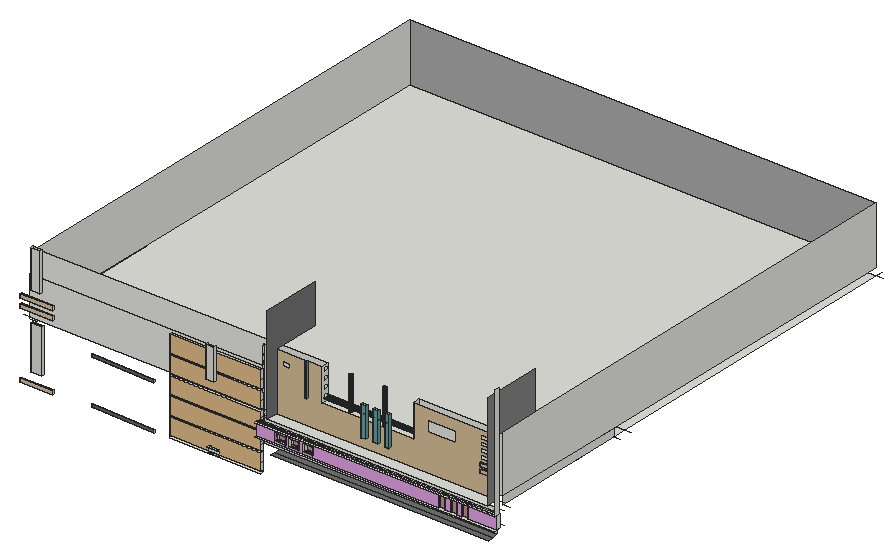
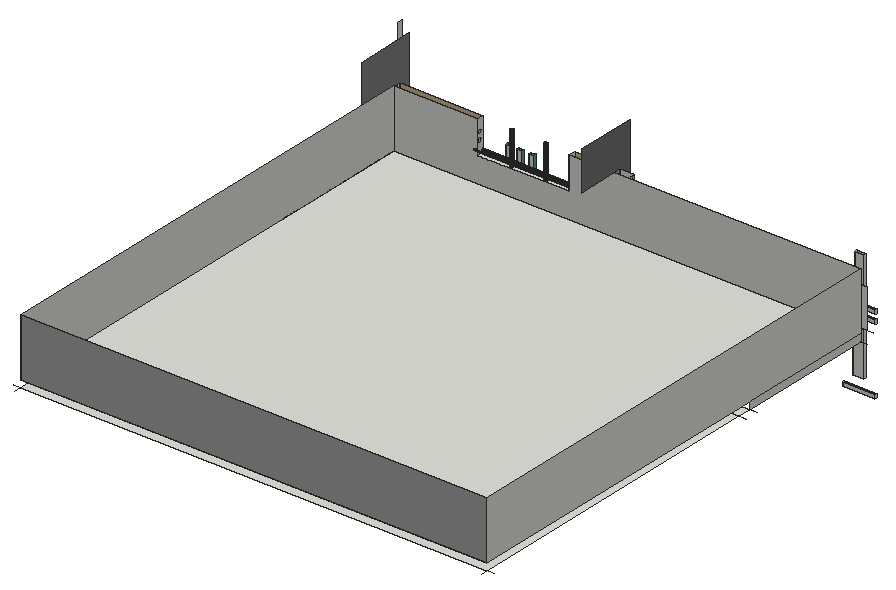
# SketchUp Ruby script. Lengths in inches.
U = 1.inch
M = Sketchup.active_model
def pt(a) = Geom::Point3d.new(a.map { |v| v * U })
def face(e, loops, mat)
  f = e.add_face(loops[0].map { |a| pt(a) })
  loops[1..].each { |l| e.add_face(l.map { |a| pt(a) }).erase! }
  f.material = f.back_material = mat if mat
  f
end
# faces: each face lists its corners as indices into pts; further lists are holes
def faces(e, pts, list, mat = nil) = list.each { |f| face(e, (f[0].is_a?(Array) ? f : [f]).map { |l| l.map { |i| pts[i] } }, mat) }
# xy, xz, yz: faces in a plane at the given z, y or x. An outline is a flat list of corners, or four numbers for a rectangle; further outlines are holes
def ring(l) = l.size == 4 ? [[l[0], l[1]], [l[2], l[1]], [l[2], l[3]], [l[0], l[3]]] : l.each_slice(2).to_a
def flat(e, list, mat, &to3) = list.each { |f| face(e, (f[0].is_a?(Array) ? f : [f]).map { |l| ring(l).map { |u, v| to3.(u, v) } }, mat) }
def xy(e, z, list, mat = nil) = flat(e, list, mat) { |x, y| [x, y, z] }
def xz(e, y, list, mat = nil) = flat(e, list, mat) { |x, z| [x, y, z] }
def yz(e, x, list, mat = nil) = flat(e, list, mat) { |y, z| [x, y, z] }
def lines(e, pts, list) = list.each { |a, b| e.add_line(pt(pts[a]), pt(pts[b])) }
# prism: a flat outline (further loops are holes) pulled along v
def prism(e, loops, v, mat = nil)
  f = face(e, loops, mat); d = Geom::Vector3d.new(v.map { |x| x * U })
  f.pushpull(f.normal.samedirection?(d) ? d.length : -d.length)
end
def box(e, o, s, mat = nil) = prism(e, [[o, [o[0] + s[0], o[1], o[2]], [o[0] + s[0], o[1] + s[1], o[2]], [o[0], o[1] + s[1], o[2]]]], [0, 0, s[2]], mat)
def at(x, y, z, deg = 0) = Geom::Transformation.translation(pt([x, y, z])) * Geom::Transformation.rotation(ORIGIN, Z_AXIS, deg.degrees)
def axes(o, x, y, z) = Geom::Transformation.new([*x, 0, *y, 0, *z, 0, *pt(o).to_a, 1])
def part(name) = M.definitions.add(name)
# library, detail: a bought-in or finely detailed component or shape, given as its bounding box
def library(name, o, s) = part(name).tap { |d| box(d.entities, o, s) }
def detail(e, o, s) = box(e.add_group.entities, o, s)
def put(e, d, t, mat = nil) = e.add_instance(d, t).tap { |i| i.material = mat if mat }
def group(e, t, mat = nil) = e.add_group.tap { |g| g.transformation = t; g.material = mat if mat }.entities
root = M.entities
M.materials.add("[0036_BurlyWood]").color = [222, 184, 135]
M.materials.add("[0042_Sienna]").color = [160, 82, 45]
M.materials.add("[0081_CadetBlue]").color = [95, 158, 160]
M.materials.add("[0119_RosyBrown]").color = [188, 143, 143]
M.materials.add("[0125_Plum]").color = [221, 160, 221]
M.materials.add("[0132_LightGray]").color = [169, 169, 169]
M.materials.add("[0133_Gray]").color = [128, 128, 128]
M.materials.add("[0134_DimGray]").color = [105, 105, 105]
M.materials.add("[Color M05]").color = [114, 114, 114]
M.materials.add("[Formica Beige]").color = [211, 187, 149]
M.materials.add("[Formica Laminate Light]").color = [213, 189, 164]
M.materials.add("[Terrazzo Tile Light]").color = [219, 217, 210]
xy(root,174.63,[[146.81,142.49,186.87,144.49]])
xy(root,178.5,[[332.83,142.31,447.24,145.31]])
xy(root,178.94,[[315.8,139.31,236.15,142.31,236.1875,143.31,315.83,140.31]])
xy(root,179.19,[[146.81,142.49,186.87,144.49]])
xy(root,180.89,[[332.83,142.31,447.24,145.31]])
xy(root,181.94,[[315.8,139.31,315.83,140.31,236.1875,143.31,236.15,142.31]])
xy(root,186.75,[[382.48,139.31,394.98,142.31]])
xy(root,191.55,[[160.7,141.49,173.95,144.49]])
xy(root,200,[[630.77,325.1,694.77,328.1]])
xy(root,201.5625,[[332.83,142.31,447.24,145.31]])
xy(root,203.95,[[332.83,142.31,447.24,145.31]])
xy(root,204,[[626.77,325.1,698.77,328.1]])
xy(root,210.6875,[[467.92,131.81,739.66,137.81],[467.92,137.81,467.92,146.81,737.81,146.81,739.66,137.81]],"[Color M05]")
xy(root,217.49,[[452.48,325.1,494.34,328.1],[494.34,325.1,497.5,328.1],[497.5,325.1,522.78,328.1],[522.78,325.1,525.94,328.1],[525.94,325.1,552.97,328.1],
  [552.97,325.1,556.13,328.1],[556.13,325.1,577.62,328.1]])
xy(root,222.93,[[447.04,325.1,583.06,328.1]])
xy(root,223.5,[[447.24,131.81,746.74,131.81,746.74,134.81,710.41,134.81,710.41,136.81,703.03,136.81,703.03,134.81,696.72,134.81,696.72,136.81,689.35,136.81,689.35,134.81,682.28,134.81,682.28,136.81,674.91,136.81,674.91,134.81,447.24,134.81],[746.74,131.81,746.81,134.81],[682.28,134.81,689.35,137.81],[696.72,134.81,703.03,137.81],[710.41,134.81,746.74,137.81],
  [746.74,134.81,746.81,137.81],[674.91,136.81,682.28,137.81],[689.35,136.81,696.72,137.81],[703.03,136.81,710.41,137.81],[674.91,137.81,682.28,139.81],
  [682.28,137.81,689.35,139.81],[689.35,137.81,696.72,139.81],[696.72,137.81,703.03,139.81],[703.03,137.81,710.41,139.81],[710.41,137.81,746.74,139.81],
  [746.74,137.81,746.81,139.81]])
xy(root,224.625,[[332.83,142.31,447.24,145.31]])
xy(root,225.72,[[470.47,134.81,483.6,137.81],[470.47,137.81,483.6,139.81]])
xy(root,225.77,[[487.65,134.81,500.68,137.81],[487.65,137.81,500.68,139.81]])
xy(root,225.82,[[504.88,134.81,517.82,137.81],[504.88,137.81,517.82,139.81]])
xy(root,226.72,[[471.48,137.81,482.6,139.81],[488.6,137.81,499.73,139.81],[505.79,137.81,516.91,139.81]])
xy(root,227.01,[[332.83,142.31,447.24,145.31]])
xy(root,234.91,[[471.48,137.81,482.6,139.81],[488.6,137.81,499.73,139.81],[505.79,137.81,516.91,139.81]])
xy(root,234.94,[[315.8,139.31,236.15,142.31,236.1875,143.31,315.83,140.31]])
xy(root,235.8125,[[504.88,134.81,517.82,137.81],[504.88,137.81,517.82,139.81]])
xy(root,235.86,[[487.65,134.81,500.68,137.81],[487.65,137.81,500.68,139.81]])
xy(root,235.91,[[470.47,134.81,483.6,137.81],[470.47,137.81,483.6,139.81]])
xy(root,237.94,[[315.8,139.31,315.83,140.31,236.1875,143.31,236.15,142.31]])
xy(root,238,[[674.91,134.81,682.28,136.81],[689.35,134.81,696.72,136.81],[703.03,134.81,710.41,136.81],[674.91,136.81,682.28,139.81],[689.35,136.81,696.72,139.81],
  [703.03,136.81,710.41,139.81]])
xy(root,240,[[447.24,131.81,737.81,134.81],[737.81,131.81,746.81,134.81],[737.81,134.81,746.81,137.81],[737.81,137.81,746.74,139.81],[746.74,137.81,746.81,139.81],
  [155.81,328.1,737.81,345.36],[155.81,345.36,737.81,737.81]])
xy(root,246.36,[[160.7,141.49,173.95,144.49]])
xy(root,247.6875,[[332.83,142.31,447.24,145.31]])
xy(root,249,[[462.98,131.81,737.83,146.81],[155.81,155.81,737.81,737.81]])
xy(root,250.08,[[332.83,142.31,447.24,145.31]])
xy(root,257.82,[[146.81,142.49,186.87,144.49]])
xy(root,261.3,[[570.73,143.81,576.42,146.81],[585.73,143.81,591.42,146.81],[599.73,143.81,605.42,146.81]])
xy(root,262.14,[[380.41,139.31,391.22,142.31]])
xy(root,262.38,[[146.81,142.49,186.87,144.49]])
xy(root,269.01,[[146.81,142.49,186.87,144.49]])
xy(root,270.75,[[332.83,142.31,447.24,145.31]])
xy(root,273.14,[[332.83,142.31,447.24,145.31],[332.83,145.31,447.24,145.43]])
xy(root,273.21,[[718.1,144.81,738.79,146.81]])
xy(root,273.57,[[146.81,142.49,186.87,144.49]])
xy(root,277.4,[[718.1,144.81,738.79,146.81]])
xy(root,279.75,[[499.64,145.31,501.58,146.81]])
xy(root,280.4375,[[[519.32,146.81,633.51,155.81],[593.46,149.88,592.9,149.99,592.39,150.23,591.95,150.6,591.625,151.07,591.43,151.61,591.39,152.18,591.49,152.74,591.74,153.26,592.11,153.69,592.58,154.02,593.11,154.21,593.68,154.25,594.24,154.15,594.76,153.91,595.19,153.54,595.52,153.07,595.71,152.53,595.76,151.96,595.65,151.4,595.41,150.88,595.04,150.45,594.57,150.12,594.03,149.93],[551.15,149.88,550.59,149.99,550.07,150.23,549.64,150.6,549.3125,151.07,549.12,151.61,549.08,152.18,549.18,152.74,549.42,153.26,549.79,153.69,550.26,154.02,550.8,154.21,551.37,154.25,551.93,154.15,552.45,153.91,552.88,153.54,553.21,153.07,553.4,152.53,553.45,151.96,553.34,151.4,553.1,150.88,552.73,150.45,552.26,150.12,551.72,149.93]],[551.15,149.88,550.59,149.99,550.07,150.23,549.64,150.6,549.3125,151.07,549.12,151.61,549.08,152.18,549.18,152.74,549.42,153.26,549.79,153.69,550.26,154.02,550.8,154.21,551.37,154.25,551.93,154.15,552.45,153.91,552.88,153.54,553.21,153.07,553.4,152.53,553.45,151.96,553.34,151.4,553.1,150.88,552.73,150.45,552.26,150.12,551.72,149.93],[593.46,149.88,592.9,149.99,592.39,150.23,591.95,150.6,591.625,151.07,591.43,151.61,591.39,152.18,591.49,152.74,591.74,153.26,592.11,153.69,592.58,154.02,593.11,154.21,593.68,154.25,594.24,154.15,594.76,153.91,595.19,153.54,595.52,153.07,595.71,152.53,595.76,151.96,595.65,151.4,595.41,150.88,595.04,150.45,594.57,150.12,594.03,149.93]])
xy(root,280.65,[[718.1,144.81,738.79,146.81]])
xy(root,282.54,[[160.41,141.49,171.66,144.49]])
xy(root,284.84,[[718.1,144.81,738.79,146.81]])
xz(root,134.81,[[[447.24,223.5,674.91,223.5,674.91,238,682.28,238,682.28,223.5,689.35,223.5,689.35,238,696.72,238,696.72,223.5,703.03,223.5,703.03,238,710.41,238,710.41,223.5,746.81,223.5,746.81,240,447.24,240],[470.47,225.72,483.6,235.91],[487.65,225.77,500.68,235.86],[504.88,225.82,517.82,235.8125]]],"[0125_Plum]")
xz(root,136.81,[[674.91,223.5,682.28,238],[689.35,223.5,696.72,238],[703.03,223.5,710.41,238]],"[0119_RosyBrown]")
xz(root,137.81,[[746.74,240,746.81,381.125]])
xz(root,137.81,[[[470.47,225.72,483.6,235.91],[471.48,226.72,482.6,234.91]],[[487.65,225.77,500.68,235.86],[488.6,226.72,499.73,234.91]],[[504.88,225.82,517.82,235.8125],[505.79,226.72,516.91,234.91]]],"[0119_RosyBrown]")
xz(root,139.31,[[380.41,262.14,391.22,300.85]],"[Terrazzo Tile Light]")
xz(root,139.81,[[674.91,223.5,682.28,238],[689.35,223.5,696.72,238],[703.03,223.5,710.41,238],[746.74,223.5,746.81,240],[[487.65,225.77,500.68,235.86],[488.6,226.72,499.73,234.91]],
  [[504.88,225.82,517.82,235.8125],[505.79,226.72,516.91,234.91]]])
xz(root,139.81,[[471.48,226.72,482.6,234.91],[488.6,226.72,499.73,234.91],[505.79,226.72,516.91,234.91]],"[0119_RosyBrown]")
xz(root,141.49,[[160.7,191.55,173.95,246.36],[160.41,282.54,171.66,330.41]],"[Terrazzo Tile Light]")
xz(root,142.31,[[382.48,178.5,394.98,180.3125],[382.48,180.3125,394.98,180.89],[382.48,180.89,394.98,184.25],[382.48,184.25,394.98,186.75],[382.48,186.75,394.98,186.8],
  [380.41,262.1,391.22,262.14],[380.41,262.14,391.22,264.58],[380.41,264.58,391.22,267.33],[380.41,267.33,391.22,270.75],[380.41,270.75,391.22,273.14]])
xz(root,142.31,[[332.83,180.89,382.48,180.89,382.48,186.8,394.98,186.8,394.98,180.89,447.24,180.89,447.24,201.5625,332.83,201.5625],[332.83,203.95,447.24,224.625],[332.83,227.01,447.24,247.6875],[332.83,250.08,447.24,250.08,447.24,270.75,391.22,270.75,391.22,262.1,380.41,262.1,380.41,270.75,332.83,270.75],[332.83,273.14,380.41,293.8125],
  [391.22,273.14,447.24,293.8125]],"[0036_BurlyWood]")
xz(root,142.49,[[146.81,174.63,186.87,179.19],[146.81,257.82,186.87,262.38],[146.81,269.01,186.87,273.57]],"[Formica Laminate Light]")
xz(root,143.81,[[570.73,261.3,576.42,298.49],[585.73,261.3,591.42,298.49],[599.73,261.3,605.42,298.49]],"[0081_CadetBlue]")
xz(root,144.49,[[146.81,174.63,186.87,179.19],[160.7,191.55,173.95,246.36],[146.81,257.82,186.87,262.38],[146.81,269.01,186.87,273.57],[160.41,282.54,171.66,330.41]])
xz(root,144.81,[[718.1,273.21,738.79,277.4],[718.1,280.65,738.79,284.84]],"[Formica Laminate Light]")
xz(root,145.31,[[332.83,180.89,447.24,201.5625],[332.83,203.95,447.24,224.625],[332.83,227.01,447.24,247.6875],[332.83,250.08,447.24,270.75],[332.83,273.14,447.24,293.8125]])
xz(root,145.31,[[332.83,178.5,447.24,180.89],[332.83,201.5625,447.24,203.95],[332.83,224.625,447.24,227.01],[332.83,247.6875,447.24,250.08],[332.83,270.75,447.24,273.14]],"[0042_Sienna]")
xz(root,145.31,[[499.64,279.75,501.58,321]],"[0081_CadetBlue]")
xz(root,145.43,[[332.83,273.14,447.24,293.8125]])
xz(root,146.81,[[447.24,210.6875,737.81,240],[155.81,249,447.24,297],[447.24,249,462.98,321],[570.73,261.3,576.42,280.4375],[585.73,261.3,591.42,280.4375],
  [599.73,261.3,605.42,280.4375],[718.1,273.21,737.83,277.4],[737.83,273.21,738.79,277.4],[499.64,279.75,500.08,321],[500.08,279.75,501.58,321],
  [570.73,280.4375,576.42,298.49],[585.73,280.4375,591.42,298.49],[599.73,280.4375,605.42,298.49],[718.1,280.65,737.83,284.84],[737.83,280.65,738.79,284.84]])
xz(root,146.81,[[[462.98,249,737.83,249,737.83,273.21,718.1,273.21,718.1,277.4,737.83,277.4,737.83,280.65,718.1,280.65,718.1,284.84,737.83,284.84,737.83,288.09,718.1,288.09,718.1,292.27,737.83,292.27,737.83,295.52,718.1,295.52,718.1,299.71,737.83,299.71,737.83,302.96,718.1,302.96,718.1,307.15,737.83,307.15,737.83,310.4,718.1,310.4,718.1,314.59,737.83,314.59,737.83,321,633.51,321,633.51,280.4375,605.42,280.4375,605.42,261.3,599.73,261.3,599.73,280.4375,591.42,280.4375,591.42,261.3,585.73,261.3,585.73,280.4375,576.42,280.4375,576.42,261.3,570.73,261.3,570.73,280.4375,519.32,280.4375,519.32,321,501.58,321,501.58,279.75,499.64,279.75,499.64,321,462.98,321],[651.72,294.73,686.34,308.41],[470.65,305.14,479.75,310.77]]],"[Formica Beige]")
xz(root,155.81,[[155.81,249,155.81,321,519.32,321,519.32,280.4375,633.51,280.4375,633.51,321,737.81,321,737.81,249]])
xz(root,737.81,[[155.81,249,737.81,321]],"[0132_LightGray]")
yz(root,146.81,[[142.49,174.63,144.49,179.19],[142.49,257.82,144.49,262.38],[142.49,269.01,144.49,273.57]])
yz(root,155.81,[[155.81,240,328.1,249],[155.81,249,737.81,321]])
yz(root,160.41,[[141.49,282.54,144.49,330.41]])
yz(root,160.7,[[141.49,191.55,144.49,246.36]])
yz(root,171.66,[[141.49,282.54,144.49,330.41]])
yz(root,173.95,[[141.49,191.55,144.49,246.36]])
yz(root,186.87,[[142.49,174.63,144.49,179.19],[142.49,257.82,144.49,262.38],[142.49,269.01,144.49,273.57]])
yz(root,332.83,[[143.31,178.5,145.31,180.89],[142.31,180.89,143.31,201.5625],[143.31,180.89,145.31,201.5625],[143.31,201.5625,145.31,203.95],[142.31,203.95,143.31,224.625],
  [143.31,203.95,145.31,224.625],[143.31,224.625,145.31,227.01],[142.31,227.01,143.31,247.6875],[143.31,227.01,145.31,247.6875],[143.31,247.6875,145.31,250.08],
  [142.31,250.08,143.31,270.75],[143.31,250.08,145.31,270.75],[143.31,270.75,145.31,273.14],[142.31,273.14,143.31,293.8125],[143.31,273.14,145.31,293.8125],
  [145.31,273.14,145.43,293.8125]])
yz(root,380.41,[[139.31,262.14,142.31,300.85]])
yz(root,391.22,[[139.31,262.14,142.31,300.85]])
yz(root,447.24,[[142.31,180.89,145.31,190.25],[142.31,190.25,145.31,201.5625],[142.31,203.95,145.31,210.6875],[142.31,210.6875,145.31,213.3125],[145.31,210.6875,146.81,223.5],
  [146.81,210.6875,148.93,223.5],[142.31,213.3125,145.31,223.5],[142.31,223.5,145.31,224.625],[145.31,223.5,146.81,240],[146.81,223.5,148.93,240],
  [142.31,227.01,145.31,236.375],[142.31,236.375,145.31,240],[142.31,240,145.31,247.6875],[145.31,240,146.81,249],[146.81,240,148.93,249],
  [145.31,249,146.81,249,146.81,319.26,145.31,319.26,145.31,293.8125,145.43,293.8125,145.43,273.14,145.31,273.14],[146.81,249,148.93,319.26],[142.31,250.08,145.31,259.4375],[142.31,259.4375,145.31,270.75],[142.31,273.14,145.31,282.5],
  [145.31,273.14,145.43,282.5],[142.31,282.5,145.31,293.8125],[145.31,282.5,145.43,293.8125]])
yz(root,462.98,[[131.81,249,146.81,249,146.81,321,206.24,321,206.24,369.72,131.81,369.72]],"[Color M05]")
yz(root,470.47,[[137.81,225.72,139.81,235.91]])
yz(root,470.47,[[134.81,225.72,137.81,235.91]],"[0119_RosyBrown]")
yz(root,471.48,[[137.81,226.72,139.81,234.91]])
yz(root,482.6,[[137.81,226.72,139.81,234.91]])
yz(root,483.6,[[134.81,225.72,137.81,235.91],[137.81,225.72,139.81,235.91]])
yz(root,487.65,[[134.81,225.77,137.81,235.86],[137.81,225.77,139.81,235.86]])
yz(root,488.6,[[137.81,226.72,139.81,234.91]])
yz(root,499.64,[[145.31,279.75,146.81,321]],"[0081_CadetBlue]")
yz(root,499.73,[[137.81,226.72,139.81,234.91]])
yz(root,500.68,[[134.81,225.77,137.81,235.86],[137.81,225.77,139.81,235.86]])
yz(root,501.58,[[145.31,279.75,146.81,321]],"[0081_CadetBlue]")
yz(root,504.88,[[134.81,225.82,137.81,235.8125],[137.81,225.82,139.81,235.8125]])
yz(root,505.79,[[137.81,226.72,139.81,234.91]])
yz(root,516.91,[[137.81,226.72,139.81,234.91]])
yz(root,517.82,[[134.81,225.82,137.81,235.8125],[137.81,225.82,139.81,235.8125]])
yz(root,519.32,[[[146.81,280.4375,155.81,321],[152.59,313.125,151.76,313.23,150.99,313.55,150.33,314.06,149.83,314.72,149.51,315.49,149.4,316.3125,149.51,317.14,149.83,317.91,150.33,318.57,150.99,319.07,151.76,319.39,152.59,319.5,153.41,319.39,154.18,319.07,154.84,318.57,155.35,317.91,155.67,317.14,155.78,316.3125,155.67,315.49,155.35,314.72,154.84,314.06,154.18,313.55,153.41,313.23],[152.59,302.8125,151.76,302.92,150.99,303.24,150.33,303.75,149.83,304.41,149.51,305.17,149.4,306,149.51,306.82,149.83,307.59,150.33,308.25,150.99,308.76,151.76,309.08,152.59,309.1875,153.41,309.08,154.18,308.76,154.84,308.25,155.35,307.59,155.67,306.82,155.78,306,155.67,305.17,155.35,304.41,154.84,303.75,154.18,303.24,153.41,302.92],[152.59,293,151.76,293.11,150.99,293.43,150.33,293.93,149.83,294.59,149.51,295.36,149.4,296.1875,149.51,297.01,149.83,297.78,150.33,298.44,150.99,298.95,151.76,299.27,152.59,299.375,153.41,299.27,154.18,298.95,154.84,298.44,155.35,297.78,155.67,297.01,155.78,296.1875,155.67,295.36,155.35,294.59,154.84,293.93,154.18,293.43,153.41,293.11],[152.59,283.0625,151.76,283.17,150.99,283.49,150.33,284,149.83,284.66,149.51,285.42,149.4,286.25,149.51,287.07,149.83,287.84,150.33,288.5,150.99,289.01,151.76,289.33,152.59,289.4375,153.41,289.33,154.18,289.01,154.84,288.5,155.35,287.84,155.67,287.07,155.78,286.25,155.67,285.42,155.35,284.66,154.84,284,154.18,283.49,153.41,283.17]]])
yz(root,570.73,[[143.81,261.3,146.81,298.49]],"[0081_CadetBlue]")
yz(root,576.42,[[143.81,261.3,146.81,298.49]],"[0081_CadetBlue]")
yz(root,585.73,[[143.81,261.3,146.81,298.49]],"[0081_CadetBlue]")
yz(root,591.42,[[143.81,261.3,146.81,298.49]],"[0081_CadetBlue]")
yz(root,599.73,[[143.81,261.3,146.81,298.49]],"[0081_CadetBlue]")
yz(root,605.42,[[143.81,261.3,146.81,298.49]],"[0081_CadetBlue]")
yz(root,633.51,[[[146.81,280.4375,155.81,321],[152.59,302.8125,153.41,302.92,154.18,303.24,154.84,303.75,155.35,304.41,155.67,305.17,155.78,306,155.67,306.82,155.35,307.59,154.84,308.25,154.18,308.76,153.41,309.08,152.59,309.1875,151.76,309.08,150.99,308.76,150.33,308.25,149.83,307.59,149.51,306.82,149.4,306,149.51,305.17,149.83,304.41,150.33,303.75,150.99,303.24,151.76,302.92],[152.59,293,153.41,293.11,154.18,293.43,154.84,293.93,155.35,294.59,155.67,295.36,155.78,296.1875,155.67,297.01,155.35,297.78,154.84,298.44,154.18,298.95,153.41,299.27,152.59,299.375,151.76,299.27,150.99,298.95,150.33,298.44,149.83,297.78,149.51,297.01,149.4,296.1875,149.51,295.36,149.83,294.59,150.33,293.93,150.99,293.43,151.76,293.11]]])
yz(root,638.57,[[152.59,283.0625,153.41,283.17,154.18,283.49,154.84,284,155.35,284.66,155.67,285.42,155.78,286.25,155.67,287.07,155.35,287.84,154.84,288.5,154.18,289.01,153.41,289.33,152.59,289.4375,151.76,289.33,150.99,289.01,150.33,288.5,149.83,287.84,149.51,287.07,149.4,286.25,149.51,285.42,149.83,284.66,150.33,284,150.99,283.49,151.76,283.17]])
yz(root,674.91,[[136.81,223.5,139.81,238]])
yz(root,674.91,[[134.81,223.5,136.81,238]],"[0119_RosyBrown]")
yz(root,682.28,[[136.81,223.5,139.81,238]])
yz(root,682.28,[[134.81,223.5,136.81,238]],"[0119_RosyBrown]")
yz(root,689.35,[[136.81,223.5,139.81,238]])
yz(root,689.35,[[134.81,223.5,136.81,238]],"[0119_RosyBrown]")
yz(root,696.72,[[136.81,223.5,139.81,238]])
yz(root,696.72,[[134.81,223.5,136.81,238]],"[0119_RosyBrown]")
yz(root,703.03,[[136.81,223.5,139.81,238]])
yz(root,703.03,[[134.81,223.5,136.81,238]],"[0119_RosyBrown]")
yz(root,710.41,[[136.81,223.5,139.81,238]])
yz(root,710.41,[[134.81,223.5,136.81,238]],"[0119_RosyBrown]")
yz(root,718.1,[[144.81,273.21,146.81,277.4],[144.81,280.65,146.81,284.84]])
yz(root,737.81,[[155.81,240,328.1,249],[155.81,249,737.81,321]])
yz(root,737.83,[[131.81,249,131.81,369.72,206.24,369.72,206.24,321,146.81,321,146.81,249]],"[0133_Gray]")
yz(root,738.79,[[144.81,273.21,146.81,277.4],[144.81,280.65,146.81,284.84]])
yz(root,746.81,[[134.81,223.5,139.81,240],[131.81,240,137.81,381.125]])
p = [[315.8,139.31,181.94],[236.15,142.31,181.94],[236.15,142.31,178.94],[315.8,139.31,178.94],[315.83,140.31,178.94],[315.83,140.31,181.94],
  [236.1875,143.31,181.94],[236.1875,143.31,178.94],[315.8,139.31,237.94],[236.15,142.31,237.94],[236.15,142.31,234.94],[315.8,139.31,234.94],
  [315.83,140.31,234.94],[315.83,140.31,237.94],[236.1875,143.31,237.94],[236.1875,143.31,234.94],[550.59,149.99,280.4375],[551.15,149.88,280.4375],
  [551.15,149.88,321.0625],[550.59,149.99,321.0625],[551.72,149.93,280.4375],[551.72,149.93,321.0625],[552.26,150.12,280.4375],[552.26,150.12,321.0625],
  [592.9,149.99,280.4375],[593.46,149.88,280.4375],[593.46,149.88,321.6875],[592.9,149.99,321.6875],[594.03,149.93,280.4375],[594.03,149.93,321.6875],
  [594.57,150.12,280.4375],[594.57,150.12,321.6875],[550.07,150.23,280.4375],[550.07,150.23,321.0625],[592.39,150.23,280.4375],[592.39,150.23,321.6875],
  [552.73,150.45,280.4375],[552.73,150.45,321.0625],[595.04,150.45,280.4375],[595.04,150.45,321.6875],[549.64,150.6,280.4375],[549.64,150.6,321.0625],
  [591.95,150.6,280.4375],[591.95,150.6,321.6875],[553.1,150.88,280.4375],[553.1,150.88,321.0625],[595.41,150.88,280.4375],[595.41,150.88,321.6875],
  [549.3125,151.07,280.4375],[549.3125,151.07,321.0625],[591.625,151.07,280.4375],[591.625,151.07,321.6875],[553.34,151.4,280.4375],[553.34,151.4,321.0625],
  [595.65,151.4,280.4375],[595.65,151.4,321.6875],[549.12,151.61,280.4375],[549.12,151.61,321.0625],[591.43,151.61,280.4375],[591.43,151.61,321.6875],
  [553.45,151.96,280.4375],[553.45,151.96,321.0625],[595.76,151.96,280.4375],[595.76,151.96,321.6875],[549.08,152.18,280.4375],[549.08,152.18,321.0625],
  [591.39,152.18,280.4375],[591.39,152.18,321.6875],[553.4,152.53,280.4375],[553.4,152.53,321.0625],[595.71,152.53,280.4375],[595.71,152.53,321.6875],
  [549.18,152.74,280.4375],[549.18,152.74,321.0625],[591.49,152.74,280.4375],[591.49,152.74,321.6875],[553.21,153.07,280.4375],[553.21,153.07,321.0625],
  [595.52,153.07,280.4375],[595.52,153.07,321.6875],[549.42,153.26,280.4375],[549.42,153.26,321.0625],[591.74,153.26,280.4375],[591.74,153.26,321.6875],
  [552.88,153.54,280.4375],[552.88,153.54,321.0625],[595.19,153.54,280.4375],[595.19,153.54,321.6875],[549.79,153.69,280.4375],[549.79,153.69,321.0625],
  [592.11,153.69,280.4375],[592.11,153.69,321.6875],[552.45,153.91,280.4375],[552.45,153.91,321.0625],[594.76,153.91,280.4375],[594.76,153.91,321.6875],
  [550.26,154.02,280.4375],[550.26,154.02,321.0625],[592.58,154.02,280.4375],[592.58,154.02,321.6875],[551.93,154.15,280.4375],[551.93,154.15,321.0625],
  [594.24,154.15,280.4375],[594.24,154.15,321.6875],[550.8,154.21,280.4375],[550.8,154.21,321.0625],[593.11,154.21,280.4375],[593.11,154.21,321.6875],
  [551.37,154.25,280.4375],[551.37,154.25,321.0625],[593.68,154.25,280.4375],[593.68,154.25,321.6875],[519.32,151.76,283.17],[519.32,152.59,283.0625],
  [638.57,152.59,283.0625],[638.57,151.76,283.17],[519.32,153.41,283.17],[638.57,153.41,283.17],[519.32,150.99,283.49],[638.57,150.99,283.49],
  [519.32,154.18,283.49],[638.57,154.18,283.49],[519.32,150.33,284],[638.57,150.33,284],[519.32,154.84,284],[638.57,154.84,284],
  [519.32,149.83,284.66],[638.57,149.83,284.66],[519.32,155.35,284.66],[638.57,155.35,284.66],[519.32,149.51,285.42],[638.57,149.51,285.42],
  [519.32,155.67,285.42],[638.57,155.67,285.42],[519.32,149.4,286.25],[638.57,149.4,286.25],[519.32,155.78,286.25],[638.57,155.78,286.25],
  [155.81,737.81,240],[155.81,746.81,240],[737.81,737.81,240],[737.81,746.81,240],[146.81,737.81,240],[155.81,345.36,240],
  [146.81,345.36,240],[155.81,328.1,240],[151.81,328.1,240],[146.81,328.1,240],[737.81,345.36,240],[746.81,345.36,240],
  [746.81,737.81,240],[737.81,328.1,240],[746.81,328.1,240],[737.81,155.81,240],[746.81,155.81,240],[155.81,155.81,240],
  [146.81,155.81,240],[155.81,146.81,249],[146.81,146.81,249],[746.81,146.81,249],[737.83,146.81,249],[737.81,139.81,240],
  [447.24,139.81,240],[737.81,146.81,223.5],[746.81,146.81,223.5],[737.81,146.81,240],[746.81,146.81,240],[737.81,137.81,240],
  [447.24,137.81,240]]
faces(root,p,[[0,1,2,3],[8,9,10,11]],"[0134_DimGray]")
faces(root,p,[[4,5,0,3],[6,5,4,7],[6,7,2,1],[12,13,8,11],[14,13,12,15],[14,15,10,9]])
faces(root,p,[[16,17,18,19],[17,20,21,18],[20,22,23,21],[24,25,26,27],[25,28,29,26],[28,30,31,29],[32,16,19,33],[34,24,27,35],
  [22,36,37,23],[30,38,39,31],[40,32,33,41],[42,34,35,43],[36,44,45,37],[38,46,47,39],[48,40,41,49],[50,42,43,51],
  [44,52,53,45],[46,54,55,47],[56,48,49,57],[58,50,51,59],[52,60,61,53],[54,62,63,55],[64,56,57,65],[66,58,59,67],
  [60,68,69,61],[62,70,71,63],[72,64,65,73],[74,66,67,75],[68,76,77,69],[70,78,79,71],[80,72,73,81],[82,74,75,83],
  [76,84,85,77],[78,86,87,79],[88,80,81,89],[90,82,83,91],[84,92,93,85],[86,94,95,87],[96,88,89,97],[98,90,91,99],
  [92,100,101,93],[94,102,103,95],[104,96,97,105],[106,98,99,107],[108,104,105,109],[100,108,109,101],[110,106,107,111],[102,110,111,103],
  [112,113,114,115],[113,116,117,114],[118,112,115,119],[116,120,121,117],[122,118,119,123],[120,124,125,121],[126,122,123,127],[124,128,129,125],
  [130,126,127,131],[128,132,133,129],[134,130,131,135],[132,136,137,133]],"[0132_LightGray]")
lines(root,p,[[138,139],[140,141],[138,142],[143,144],[145,146],[146,147],[148,149],[140,150],[151,152],[153,154],[155,156],[157,158],
  [159,160],[161,162],[163,164],[165,166],[167,168]])
